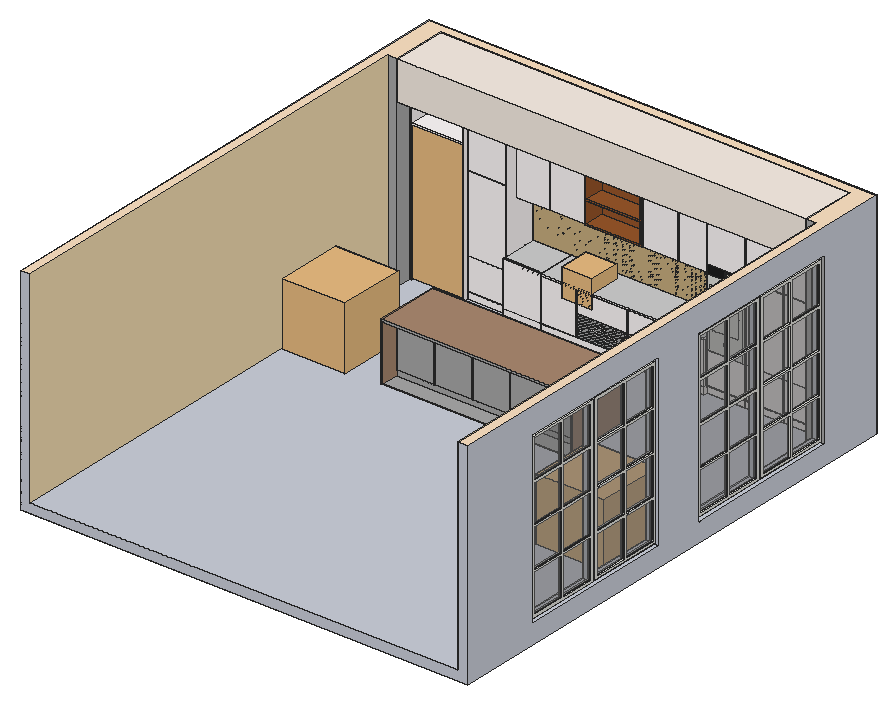
# SketchUp Ruby script. Lengths in millimetres.
U = 1.mm
M = Sketchup.active_model
def pt(a) = Geom::Point3d.new(a.map { |v| v * U })
def face(e, loops, mat)
  f = e.add_face(loops[0].map { |a| pt(a) })
  loops[1..].each { |l| e.add_face(l.map { |a| pt(a) }).erase! }
  f.material = f.back_material = mat if mat
  f
end
# faces: each face lists its corners as indices into pts; further lists are holes
def faces(e, pts, list, mat = nil) = list.each { |f| face(e, (f[0].is_a?(Array) ? f : [f]).map { |l| l.map { |i| pts[i] } }, mat) }
# xy, xz, yz: faces in a plane at the given z, y or x. An outline is a flat list of corners, or four numbers for a rectangle; further outlines are holes
def ring(l) = l.size == 4 ? [[l[0], l[1]], [l[2], l[1]], [l[2], l[3]], [l[0], l[3]]] : l.each_slice(2).to_a
def flat(e, list, mat, &to3) = list.each { |f| face(e, (f[0].is_a?(Array) ? f : [f]).map { |l| ring(l).map { |u, v| to3.(u, v) } }, mat) }
def xy(e, z, list, mat = nil) = flat(e, list, mat) { |x, y| [x, y, z] }
def xz(e, y, list, mat = nil) = flat(e, list, mat) { |x, z| [x, y, z] }
def yz(e, x, list, mat = nil) = flat(e, list, mat) { |y, z| [x, y, z] }
def lines(e, pts, list) = list.each { |a, b| e.add_line(pt(pts[a]), pt(pts[b])) }
# prism: a flat outline (further loops are holes) pulled along v
def prism(e, loops, v, mat = nil)
  f = face(e, loops, mat); d = Geom::Vector3d.new(v.map { |x| x * U })
  f.pushpull(f.normal.samedirection?(d) ? d.length : -d.length)
end
def box(e, o, s, mat = nil) = prism(e, [[o, [o[0] + s[0], o[1], o[2]], [o[0] + s[0], o[1] + s[1], o[2]], [o[0], o[1] + s[1], o[2]]]], [0, 0, s[2]], mat)
def at(x, y, z, deg = 0) = Geom::Transformation.translation(pt([x, y, z])) * Geom::Transformation.rotation(ORIGIN, Z_AXIS, deg.degrees)
def axes(o, x, y, z) = Geom::Transformation.new([*x, 0, *y, 0, *z, 0, *pt(o).to_a, 1])
def part(name) = M.definitions.add(name)
# library, detail: a bought-in or finely detailed component or shape, given as its bounding box
def library(name, o, s) = part(name).tap { |d| box(d.entities, o, s) }
def detail(e, o, s) = box(e.add_group.entities, o, s)
def put(e, d, t, mat = nil) = e.add_instance(d, t).tap { |i| i.material = mat if mat }
def group(e, t, mat = nil) = e.add_group.tap { |g| g.transformation = t; g.material = mat if mat }.entities
root = M.entities
M.materials.add("[0009_Linen]").color = [250, 240, 230]
M.materials.add("[0010_Snow]").color = [255, 250, 250]
M.materials.add("[0012_Bisque]").color = [255, 228, 196]
M.materials.add("[0034_Wheat]").color = [245, 222, 179]
M.materials.add("[0132_LightGray]").color = [169, 169, 169]
M.materials.add("[Carrera Marble]").color = [207, 207, 207]
M.materials.add("[Color M03]").color = [170, 170, 170]
M.materials.add("[Color_008]").color = [30, 30, 30]
M.materials.add("[Marble Carrara Floor Tile]").color = [204, 208, 219]
M.materials.add("[Roofing Slate Tan]").color = [200, 175, 128]
M.materials.add("[Tile Veriegated Stone]").color = [171, 137, 112]
M.materials.add("[Translucent Glass Gray]").color = [128, 128, 128]
M.materials["[Translucent Glass Gray]"].alpha = 0.5
M.materials.add("[Wood Cherry Original]").color = [152, 86, 42]
c1 = library("Untitled",[1978.1,21049.9,34.3],[1077.2,950.8,1997.1])
c2 = library("Component_3",[0,0,0],[480,480,433.8])
c3 = part("kg")
xy(c3.entities,0.03,[[[6.76,0,6.01,0.06,5.3,0.21,5.3,1.09,5.35,1.09,5.6,0.99,5.97,0.88,6.4,0.79,6.83,0.75,7.19,0.78,7.49,0.85,7.73,0.98,7.91,1.14,8.11,1.56,8.17,2.11,8.17,2.55,7.83,2.3,7.51,2.12,7.14,2.01,6.69,1.98,6.28,2.02,5.92,2.13,5.6,2.33,5.33,2.61,5.11,2.96,4.95,3.38,4.85,3.87,4.82,4.43,4.87,5.02,5,5.54,5.2,5.98,5.47,6.35,5.77,6.64,6.13,6.85,6.52,6.98,6.93,7.02,7.6,6.93,8.17,6.67,8.22,6.88,9.01,6.88,9.01,2.46,8.98,1.87,8.87,1.36,8.7,0.93,8.46,0.59,8.14,0.33,7.76,0.15,7.3,0.04],[6.87,2.75,7.21,2.79,7.55,2.88,7.88,3.04,8.17,3.25,8.17,5.99,7.59,6.2,7.06,6.27,6.76,6.24,6.49,6.15,6.26,6,6.06,5.8,5.9,5.54,5.78,5.23,5.69,4.45,5.76,3.72,5.97,3.19,6.13,3,6.34,2.86,6.58,2.78]],[0.61,1.89,0.61,8.85,1.45,8.85,1.45,4.77,3.42,6.88,4.47,6.88,2.42,4.8,4.75,1.89,3.64,1.89,1.78,4.3,1.45,3.98,1.45,1.89]])
c4 = part("12:15")
xy(c4.entities,0.1,[[2.4,0,2.1,0.1,1.9,0.2,1.7,0.4,1.7,1,1.9,1.2,2.1,1.3,2.4,1.4,4.5,1.4,4.5,9.6,2.1,9.6,1.7,10,1.7,10.6,1.9,10.8,2.1,10.9,2.4,11,5.9,11,5.9,1.4,7.3,1.4,7.3,4.6,7.5,4.8,7.7,4.9,8,5,8.2,4.9,8.5,4.8,8.6,4.6,8.7,4.3,8.7,0.7,8.6,0.4,8.5,0.2,8.2,0.1,8,0],[11.9,0,11.9,4.8,12,5.3,12.3,5.8,12.8,6.1,13.3,6.2,17.5,6.2,17.5,9.6,12.3,9.6,11.9,10,11.9,10.6,12.1,10.8,12.3,10.9,12.6,11,17.5,11,18.1,10.9,18.5,10.6,18.9,10.1,19,9.6,19,6.2,18.9,5.7,18.5,5.2,18.1,4.9,17.5,4.8,13.3,4.8,13.3,1.4,18.3,1.4,18.7,1.2,18.9,1,19,0.7,18.9,0.4,18.7,0.2,18.3,0],[33.1,0,32.8,0.1,32.6,0.2,32.4,0.4,32.4,1,32.6,1.2,32.8,1.3,33.1,1.4,35.2,1.4,35.2,9.6,32.8,9.6,32.6,9.8,32.5,10,32.4,10.3,32.5,10.6,32.6,10.8,32.8,10.9,33.1,11,36.6,11,36.6,1.4,38,1.4,38,4.6,38.2,4.8,38.4,4.9,38.7,5,39,4.9,39.2,4.8,39.3,4.6,39.4,4.3,39.4,0.7,39.3,0.4,39.2,0.2,39,0.1,38.7,0],[45.2,0,44.8,0.1,44.3,0.2,43.2,0.6,42.9,0.9,42.8,1.3,42.9,1.6,43,1.8,43.2,2,43.5,2,44,1.9,44.9,1.5,45.2,1.4,48.4,1.4,48.4,4.8,44.2,4.8,44.2,11,49.1,11,49.4,10.9,49.6,10.8,49.8,10.6,49.8,10,49.4,9.6,45.6,9.6,45.6,6.2,48.4,6.2,49,6.1,49.4,5.8,49.7,5.3,49.8,4.8,49.8,1.4,49.7,0.9,49.4,0.4,49,0.1,48.4,0],[24.7,1.8,24.3,2.2,24.3,3.9,24.5,4.2,24.7,4.3,25,4.4,26.4,4.4,26.6,4.3,26.9,4.2,27,3.9,27.1,3.7,27.1,2.5,27,2.2,26.9,2,26.7,1.8],
  [24.7,6.6,24.3,7,24.3,8.7,24.5,9,24.7,9.1,25,9.2,26.4,9.2,26.7,9.1,26.9,8.9,27.1,8.5,27.1,7.3,27,7,26.9,6.8,26.7,6.6]])
c5 = part("Siemens")
xy(c5.entities,0.1,[[3.5,0,2.8,0.1,2.2,0.6,1.8,1.2,1.7,1.8,1.7,2.2,1.9,2.4,2.1,2.5,2.4,2.6,2.7,2.5,2.9,2.4,3.1,2.2,3.1,1.7,3.4,1.4,7.3,1.4,7.3,1.6,7.2,1.8,2.1,8.4,1.8,8.9,1.7,9.4,1.8,10,2.2,10.5,2.7,10.9,3.3,11,6.9,11,7.5,10.9,8.2,10.4,8.6,9.8,8.7,9.1,8.7,8.8,8.3,8.4,7.8,8.4,7.6,8.5,7.1,9.5,6.8,9.6,3.4,9.6,3.2,9.5,3.1,9.4,3.2,9.2,8.4,2.6,8.7,2.1,8.7,1.6,8.6,1,8.3,0.5,7.8,0.1,7.3,0],[13.3,0,13.1,0.1,12.8,0.2,12.7,0.4,12.6,0.7,12.7,1,12.8,1.2,13.1,1.4,14.7,1.4,14.7,6.6,13.1,6.6,12.8,6.8,12.7,7,12.6,7.3,12.7,7.6,12.8,7.8,13.1,8,15.7,8,16,7.8,16.1,7.6,16.2,7.3,16.2,1.4,17.8,1.4,18.2,1,18.3,0.7,18.2,0.4,18.1,0.2,17.8,0.1,17.6,0],[[24.8,0,24.1,0.2,23.5,0.5,22.9,1,22.6,1.3,22.2,2.1,22.2,5.6,22.4,6.3,22.6,6.8,22.9,7.1,24.1,7.9,24.8,8,26.7,8,27.4,7.8,28.1,7.4,28.9,6.6,29.1,6.2,29.2,5.4,29.2,3.7,29.1,3.4,29,3.2,28.8,3,23.6,3,23.6,2.6,23.7,2.3,23.9,2,24.3,1.6,24.9,1.4,28.5,1.4,28.8,1.3,29,1.2,29.1,1,29.2,0.7,29.1,0.4,29,0.2,28.8,0.1,28.5,0],[23.6,4.4,27.8,4.4,27.8,5.7,27.6,6,27.2,6.3,26.9,6.5,26.6,6.6,24.9,6.6,24.3,6.4,23.7,5.8,23.6,5.5]],[33,0,32.7,0.1,32.5,0.2,32.3,0.4,32.3,7.6,32.5,7.8,32.7,7.9,33,8,33.4,7.9,33.6,7.5,34.2,7.9,34.9,8,35.3,8,35.7,7.8,36,7.6,36.3,7.3,37,7.8,37.4,8,37.7,8,38.3,7.9,38.9,7.5,39.2,7,39.4,6.4,39.6,0.7,39.5,0.4,39.4,0.2,39.1,0.1,38.9,0,38.6,0.1,38.4,0.2,38.2,0.4,38.2,0.7,38,6.1,37.9,6.5,37.7,6.6,37.4,6.5,36.6,5.8,36.6,0.4,36.4,0.2,36.2,0.1,35.9,0,35.7,0.1,35.4,0.2,35.3,0.4,35.2,0.7,35.2,6.2,35.1,6.5,34.9,6.6,34.6,6.5,33.6,5.6,33.6,0.4,33.4,0.2],[[45.3,0,44.5,0.2,44,0.5,43.3,1,43.1,1.3,42.8,1.7,42.7,2.1,42.7,5.6,42.9,6.3,43.1,6.8,43.4,7.1,44.6,7.9,45.2,8,47.2,8,47.9,7.8,48.6,7.4,49.4,6.6,49.7,5.4,49.7,3.7,49.6,3.4,49.5,3.2,49.2,3,44.1,3,44.1,2.3,44.8,1.6,45.4,1.4,49,1.4,49.2,1.3,49.5,1.2,49.6,1,49.7,0.7,49.6,0.4,49.5,0.2,49.2,0.1,49,0],[44.1,4.4,48.3,4.4,48.3,5.4,48.1,6,47.7,6.3,47.4,6.5,47.1,6.6,45.3,6.6,45,6.5,44.8,6.4,44.3,6,44.1,5.8]],
  [53.6,0,53.3,0.1,53.1,0.2,53,0.4,52.9,0.7,52.9,7.3,53,7.6,53.1,7.8,53.3,8,53.9,8,54.1,7.8,54.2,7.6,54.3,7.3,54.3,6.8,55.6,7.6,56.2,7.9,57,8,57.7,8,58.4,7.9,59.1,7.4,59.6,6.8,59.7,6,59.9,0.7,59.9,0.4,59.7,0.2,59.5,0.1,59.2,0,59,0,58.7,0.2,58.6,0.4,58.5,0.7,58.3,5.9,58.3,6.2,57.9,6.6,56.5,6.6,56.2,6.4,54.3,5.1,54.3,0.7,54.2,0.4,54.1,0.2,53.9,0.1],[65.1,0,64.4,0.1,63.8,0.4,63.3,0.9,63.1,1.3,63.2,1.5,63.3,1.8,63.9,2,64.1,1.9,64.4,1.7,64.8,1.5,65.3,1.4,68.2,1.4,68.4,1.6,68.6,1.9,68.6,2.2,68.5,2.6,68.1,2.8,64.4,4.5,63.9,4.8,63.6,5.2,63.4,5.7,63.3,6.1,63.4,6.8,63.8,7.4,64.4,7.9,65.1,8,68.3,8,69,7.9,69.6,7.5,70,7.1,70.2,6.7,70.1,6.4,70,6.2,69.7,6,69.5,6,69.2,6.1,68.6,6.5,68.3,6.6,65.2,6.6,64.8,6.5,64.7,6.2,64.8,6,65,5.8,68.7,4.2,69.2,3.8,69.6,3.4,69.9,2.8,70,2.1,69.8,1.3,69.6,0.9,69.4,0.6,68.7,0.2,67.9,0],[14.7,9.6,14.4,9.7,14.2,9.8,14.1,10.1,14,10.3,14,10.9,14.1,11.2,14.2,11.4,14.5,11.6,15.7,11.6,16,11.4,16.1,11.2,16.2,10.9,16.2,10.3,16.1,10.1,16,9.8,15.7,9.7,15.5,9.6]])
c6 = part("Naamloos")
xy(c6.entities,0,[[0,-594,550,0]])
xy(c6.entities,304,[[-14,-534,0,-514],[-14,-80,0,-60]])
xy(c6.entities,324,[[-14,-534,0,-514],[-14,-80,0,-60]])
xy(c6.entities,367.3,[[-3,-350,0,-333.4],[-3,-333.4,0,-316.8],[-3,-316.8,0,-302.6],[-3,-302.6,0,-286.7],[-3,-286.7,0,-271.3],
  [-3,-271.3,0,-257.1],[-3,-257.1,0,-244]])
xy(c6.entities,375.3,[[-3,-350,0,-333.4],[-3,-333.4,0,-316.8],[-3,-316.8,0,-302.6],[-3,-302.6,0,-286.7],[-3,-286.7,0,-271.3],
  [-3,-271.3,0,-257.1],[-3,-257.1,0,-244]])
xy(c6.entities,450,[[0,-594,550,0]])
xz(c6.entities,-594,[[0,0,550,450]])
xz(c6.entities,-534,[[-14,304,-11.4,304.3,-9,305.3,-6.9,306.9,-5.3,309,-4.3,311.4,-4,314,-4.3,316.6,-5.3,319,-6.9,321.1,-9,322.7,-11.4,323.7,-14,324,-16.6,323.7,-19,322.7,-21.1,321.1,-22.7,319,-23.7,316.6,-24,314,-23.7,311.4,-22.7,309,-21.1,306.9,-19,305.3,-16.6,304.3],[-14,304,0,324]])
xz(c6.entities,-514,[[-14,304,0,324]])
xz(c6.entities,-350,[[-3,367.3,0,375.3]])
xz(c6.entities,-244,[[-3,367.3,0,375.3]])
xz(c6.entities,-80,[[-14,304,0,324]])
xz(c6.entities,-60,[[-14,304,-16.6,304.3,-19,305.3,-21.1,306.9,-22.7,309,-23.7,311.4,-24,314,-23.7,316.6,-22.7,319,-21.1,321.1,-19,322.7,-16.6,323.7,-14,324,-11.4,323.7,-9,322.7,-6.9,321.1,-5.3,319,-4.3,316.6,-4,314,-4.3,311.4,-5.3,309,-6.9,306.9,-9,305.3,-11.4,304.3],[-14,304,0,324]])
xz(c6.entities,0,[[0,0,550,450]])
yz(c6.entities,-14,[[-534,304,-514,324],[-80,304,-60,324]])
yz(c6.entities,-6,[[-388.4,353.6,-392.8,354.2,-396.9,356,-400.3,358.7,-403,362.3,-404.6,366.4,-405.1,370.8,-404.5,375.2,-402.7,379.3,-399.9,382.8,-396.4,385.4,-392.2,387,-387.8,387.5,-383.4,386.9,-379.4,385.1,-375.9,382.4,-373.2,378.8,-371.6,374.7,-371.1,370.3,-371.8,365.9,-373.5,361.8,-376.3,358.3,-379.9,355.7,-384,354.1],[-206.2,354.2,-210.9,354.3,-215.4,355.7,-219.4,358.1,-222.7,361.6,-224.9,365.7,-226,370.3,-225.8,375,-224.5,379.5,-222,383.5,-218.6,386.7,-214.5,388.9,-209.9,390,-205.2,389.9,-200.7,388.5,-196.7,386.1,-193.5,382.6,-191.2,378.5,-190.2,373.9,-190.3,369.2,-191.6,364.7,-194.1,360.7,-197.5,357.5,-201.7,355.3]])
yz(c6.entities,-3,[[-350,367.3,-333.4,375.3],[-333.4,367.3,-316.8,375.3],[-316.8,367.3,-302.6,375.3],[-302.6,367.3,-286.7,375.3],[-286.7,367.3,-271.3,375.3],
  [-271.3,367.3,-257.1,375.3],[-257.1,367.3,-244,375.3]])
yz(c6.entities,0,[[[-594,0,-594,400,0,400,0,0,-30,0,-30,350,-564,350,-564,0],[-206.2,354.2,-201.7,355.3,-197.5,357.5,-194.1,360.7,-191.6,364.7,-190.3,369.2,-190.2,373.9,-191.2,378.5,-193.5,382.6,-196.7,386.1,-200.7,388.5,-205.2,389.9,-209.9,390,-214.5,388.9,-218.6,386.7,-222,383.5,-224.5,379.5,-225.8,375,-226,370.3,-224.9,365.7,-222.7,361.6,-219.4,358.1,-215.4,355.7,-210.9,354.3],[-388.4,353.6,-384,354.1,-379.9,355.7,-376.3,358.3,-373.5,361.8,-371.8,365.9,-371.1,370.3,-371.6,374.7,-373.2,378.8,-375.9,382.4,-379.4,385.1,-383.4,386.9,-387.8,387.5,-392.2,387,-396.4,385.4,-399.9,382.8,-402.7,379.3,-404.5,375.2,-405.1,370.8,-404.6,366.4,-403,362.3,-400.3,358.7,-396.9,356,-392.8,354.2],[-350,367.3,-244,375.3],[-249.2,382.1,-248.5,382.2,-247.7,382.5,-247.1,383,-246.6,383.6,-246.3,384.3,-246.2,385.1,-246.3,385.9,-246.6,386.6,-247.1,387.2,-247.7,387.7,-248.5,388,-249.2,388.1,-250,388,-250.7,387.7,-251.4,387.2,-251.8,386.6,-252.1,385.9,-252.2,385.1,-252.1,384.3,-251.8,383.6,-251.4,383,-250.7,382.5,-250,382.2],[-309.9,381.3,-309.1,381.4,-308.4,381.7,-307.8,382.1,-307.3,382.8,-307,383.5,-306.9,384.3,-307,385,-307.3,385.8,-307.8,386.4,-308.4,386.9,-309.1,387.2,-309.9,387.3,-310.7,387.2,-311.4,386.9,-312,386.4,-312.5,385.8,-312.8,385,-312.9,384.3,-312.8,383.5,-312.5,382.8,-312,382.1,-311.4,381.7,-310.7,381.4]],[[-564,0,-30,350],[-497,113,-97,263],[-534,304,-514,324],[-80,304,-60,324]],[-497,113,-97,263],[-309.9,381.3,-310.7,381.4,-311.4,381.7,-312,382.1,-312.5,382.8,-312.8,383.5,-312.9,384.3,-312.8,385,-312.5,385.8,-312,386.4,-311.4,386.9,-310.7,387.2,-309.9,387.3,-309.1,387.2,-308.4,386.9,-307.8,386.4,-307.3,385.8,-307,385,-306.9,384.3,-307,383.5,-307.3,382.8,-307.8,382.1,-308.4,381.7,-309.1,381.4],[-249.2,382.1,-250,382.2,-250.7,382.5,-251.4,383,-251.8,383.6,-252.1,384.3,-252.2,385.1,-252.1,385.9,-251.8,386.6,-251.4,387.2,-250.7,387.7,-250,388,-249.2,388.1,-248.5,388,-247.7,387.7,-247.1,387.2,-246.6,386.6,-246.3,385.9,-246.2,385.1,-246.3,384.3,-246.6,383.6,-247.1,383,-247.7,382.5,-248.5,382.2]])
yz(c6.entities,0,[[-594,400,0,450]],"[Color_008]")
yz(c6.entities,550,[[-594,0,0,450]])
p = [[-14,-534,304],[-16.6,-534,304.3],[-16.6,-60,304.3],[-14,-60,304],[-14,-80,304],[-11.4,-534,304.3],
  [-11.4,-60,304.3],[-19,-534,305.3],[-19,-60,305.3],[-9,-534,305.3],[-9,-60,305.3],[-21.1,-534,306.9],
  [-21.1,-60,306.9],[-6.9,-534,306.9],[-6.9,-60,306.9],[-22.7,-534,309],[-22.7,-60,309],[-5.3,-534,309],
  [-5.3,-60,309],[-23.7,-534,311.4],[-23.7,-60,311.4],[-4.3,-534,311.4],[-4.3,-60,311.4],[-24,-534,314],
  [-24,-60,314],[-4,-534,314],[-4,-60,314],[-23.7,-534,316.6],[-23.7,-60,316.6],[-4.3,-534,316.6],
  [-4.3,-60,316.6],[-22.7,-534,319],[-22.7,-60,319],[-5.3,-534,319],[-5.3,-60,319],[-21.1,-534,321.1],
  [-21.1,-60,321.1],[-6.9,-534,321.1],[-6.9,-60,321.1],[-19,-534,322.7],[-19,-60,322.7],[-9,-534,322.7],
  [-9,-60,322.7],[-16.6,-534,323.7],[-16.6,-60,323.7],[-11.4,-534,323.7],[-11.4,-60,323.7],[-14,-534,324],
  [-14,-80,324],[-14,-60,324],[0,-388.4,353.6],[0,-392.8,354.2],[-6,-392.8,354.2],[-6,-388.4,353.6],
  [0,-384,354.1],[-6,-384,354.1],[0,-379.9,355.7],[-6,-379.9,355.7],[0,-396.9,356],[-6,-396.9,356],
  [0,-206.2,354.2],[0,-210.9,354.3],[-6,-210.9,354.3],[-6,-206.2,354.2],[0,-201.7,355.3],[-6,-201.7,355.3],
  [0,-215.4,355.7],[-6,-215.4,355.7],[0,-197.5,357.5],[-6,-197.5,357.5],[0,-376.3,358.3],[-6,-376.3,358.3],
  [0,-219.4,358.1],[-6,-219.4,358.1],[0,-400.3,358.7],[-6,-400.3,358.7],[0,-194.1,360.7],[-6,-194.1,360.7],
  [0,-222.7,361.6],[-6,-222.7,361.6],[0,-373.5,361.8],[-6,-373.5,361.8],[0,-403,362.3],[-6,-403,362.3],
  [0,-191.6,364.7],[-6,-191.6,364.7],[0,-224.9,365.7],[-6,-224.9,365.7],[0,-371.8,365.9],[-6,-371.8,365.9],
  [0,-404.6,366.4],[-6,-404.6,366.4],[0,-190.3,369.2],[-6,-190.3,369.2],[0,-226,370.3],[-6,-226,370.3],
  [0,-371.1,370.3],[-6,-371.1,370.3],[0,-405.1,370.8],[-6,-405.1,370.8],[0,-190.2,373.9],[-6,-190.2,373.9],
  [0,-371.6,374.7],[-6,-371.6,374.7],[0,-225.8,375],[-6,-225.8,375],[0,-404.5,375.2],[-6,-404.5,375.2],
  [0,-191.2,378.5],[-6,-191.2,378.5],[0,-373.2,378.8],[-6,-373.2,378.8],[0,-224.5,379.5],[-6,-224.5,379.5],
  [0,-402.7,379.3],[-6,-402.7,379.3],[0,-193.5,382.6],[-6,-193.5,382.6],[0,-375.9,382.4],[-6,-375.9,382.4],
  [0,-399.9,382.8],[-6,-399.9,382.8],[0,-222,383.5],[-6,-222,383.5],[0,-379.4,385.1],[-6,-379.4,385.1],
  [0,-196.7,386.1],[-6,-196.7,386.1],[0,-396.4,385.4],[-6,-396.4,385.4],[0,-218.6,386.7],[-6,-218.6,386.7],
  [0,-383.4,386.9],[-6,-383.4,386.9],[0,-392.2,387],[-6,-392.2,387],[0,-200.7,388.5],[-6,-200.7,388.5],
  [0,-214.5,388.9],[-6,-214.5,388.9],[0,-387.8,387.5],[-6,-387.8,387.5],[0,-205.2,389.9],[-6,-205.2,389.9],
  [0,-209.9,390],[-6,-209.9,390],[0,-260.1,384.4],[0,-266.1,384.4],[0,-275.9,384.4],[0,-281.9,384.4],
  [0,-279.1,381.9],[0,-279.1,386.9],[0,-309.9,387.3],[0,-309.9,384.3],[0,-307.9,384.3]]
faces(c6.entities,p,[[0,1,2,3,4],[5,0,4,3,6],[1,7,8,2],[9,5,6,10],[7,11,12,8],[13,9,10,14],[11,15,16,12],[17,13,14,18],
  [15,19,20,16],[21,17,18,22],[19,23,24,20],[25,21,22,26],[23,27,28,24],[29,25,26,30],[27,31,32,28],[33,29,30,34],
  [31,35,36,32],[37,33,34,38],[35,39,40,36],[41,37,38,42],[39,43,44,40],[45,41,42,46],[43,47,48,49,44],[47,45,46,49,48],
  [50,51,52,53],[54,50,53,55],[56,54,55,57],[51,58,59,52],[60,61,62,63],[64,60,63,65],[61,66,67,62],[68,64,65,69],
  [70,56,57,71],[66,72,73,67],[58,74,75,59],[76,68,69,77],[72,78,79,73],[80,70,71,81],[74,82,83,75],[84,76,77,85],
  [78,86,87,79],[88,80,81,89],[82,90,91,83],[92,84,85,93],[86,94,95,87],[96,88,89,97],[90,98,99,91],[100,92,93,101],
  [102,96,97,103],[94,104,105,95],[98,106,107,99],[108,100,101,109],[110,102,103,111],[104,112,113,105],[106,114,115,107],[116,108,109,117],
  [118,110,111,119],[114,120,121,115],[112,122,123,113],[124,118,119,125],[126,116,117,127],[120,128,129,121],[122,130,131,123],[132,124,125,133],
  [128,134,135,129],[136,126,127,137],[130,138,139,131],[140,132,133,141],[134,140,141,135],[142,136,137,143],[138,144,145,139],[144,142,143,145]])
lines(c6.entities,p,[[146,147],[148,149],[150,151],[152,153],[153,154]])
put(c6.entities,c3,axes([0,-289.7,380.2],[0,-1,0],[0,0,1],[-1,0,0]))
put(c6.entities,c4,axes([0,-270.7,426.7],[0,-1,0],[0,0,1],[-1,0,0]))
put(c6.entities,c5,axes([0,-261.9,52.3],[0,-1,0],[0,0,1],[-1,0,0]))
c7 = library("plant",[-542,-691.1,-9.7],[1064.4,1045.2,990])
xy(root,890,[[2650,7330,3150,7730]])
xy(root,900,[[2650,7330,3150,7730]])
xy(root,910,[[2650,7330,3150,7730]])
xy(root,920,[[[2650,7330,3150,7730],[2677.7,7357.7,3122.3,7702.3]],[2677.7,7357.7,3122.3,7702.3]])
xy(root,950,[[1750.2,7850,4900,8510]])
xy(root,1700,[[1750.2,7850,4900,8510]])
xz(root,7250,[[2900,250,4300,585]],"[Color M03]")
xz(root,7330,[[2650,890,3150,900],[2650,900,3150,910],[2650,910,3150,920]])
xz(root,7730,[[2650,890,3150,900],[2650,900,3150,910],[2650,910,3150,920]])
xz(root,7850,[[1750.2,950,4900,1700]],"[Roofing Slate Tan]")
xz(root,8510,[[1750.2,950,4900,1700]])
yz(root,1750.2,[[7850,950,8510,1700]])
yz(root,2650,[[7330,890,7730,900],[7330,900,7730,910],[7330,910,7730,920]])
yz(root,3150,[[7330,890,7730,900],[7330,900,7730,910],[7330,910,7730,920]])
yz(root,4900,[[7850,950,8510,1700]])
p = [[1750,7250,250],[2350,7250,250]]
lines(root,p,[[0,1]])
put(root,c1,axes([-1257.1,-2186.7,142.2],[0.77804,0,0],[0,0.4483,0],[0,0,1.07208]))
put(root,c2,at(2670,7730,721.8,-90))
put(root,c6,axes([4901,7310,755],[0,0.57,0],[-1,0,0],[0,0,2.66667]))
put(root,c7,at(621.6,5612.8,150))
put(root,c7,at(6172.1,3743.6,159.7))
g1 = group(root,at(6925,4550,350))
xy(g1,0,[[0,-3250,50,-2075],[0,-2025,50,-850],[0,0,50,1175]])
xy(g1,30,[[0,-3220,30,-2672.5],[30,-3220,50,-2672.5],[0,-2652.5,30,-2105],[30,-2652.5,50,-2105],[0,-1995,30,-1447.5],
  [30,-1995,50,-1447.5],[0,-1427.5,30,-880],[30,-1427.5,50,-880],[0,30,30,577.5],[30,30,50,577.5],
  [0,597.5,30,1145],[30,597.5,50,1145]])
xy(g1,637.5,[[0,-3220,30,-2672.5],[30,-3220,50,-2672.5],[0,-2652.5,30,-2105],[30,-2652.5,50,-2105],[0,-1995,30,-1447.5],
  [30,-1995,50,-1447.5],[0,-1427.5,30,-880],[30,-1427.5,50,-880],[0,30,30,577.5],[30,30,50,577.5],
  [0,597.5,30,1145],[30,597.5,50,1145]])
xy(g1,657.5,[[0,-3220,30,-2672.5],[30,-3220,50,-2672.5],[0,-2652.5,30,-2105],[30,-2652.5,50,-2105],[0,-1995,30,-1447.5],
  [30,-1995,50,-1447.5],[0,-1427.5,30,-880],[30,-1427.5,50,-880],[0,30,30,577.5],[30,30,50,577.5],
  [0,597.5,30,1145],[30,597.5,50,1145]])
xy(g1,1265,[[0,-3220,30,-2672.5],[30,-3220,50,-2672.5],[0,-2652.5,30,-2105],[30,-2652.5,50,-2105],[0,-1995,30,-1447.5],
  [30,-1995,50,-1447.5],[0,-1427.5,30,-880],[30,-1427.5,50,-880],[0,30,30,577.5],[30,30,50,577.5],
  [0,597.5,30,1145],[30,597.5,50,1145]])
xy(g1,1285,[[0,-3220,30,-2672.5],[30,-3220,50,-2672.5],[0,-2652.5,30,-2105],[30,-2652.5,50,-2105],[0,-1995,30,-1447.5],
  [30,-1995,50,-1447.5],[0,-1427.5,30,-880],[30,-1427.5,50,-880],[0,30,30,577.5],[30,30,50,577.5],
  [0,597.5,30,1145],[30,597.5,50,1145]])
xy(g1,1892.5,[[0,-3220,30,-2672.5],[30,-3220,50,-2672.5],[0,-2652.5,30,-2105],[30,-2652.5,50,-2105],[0,-1995,30,-1447.5],
  [30,-1995,50,-1447.5],[0,-1427.5,30,-880],[30,-1427.5,50,-880],[0,30,30,577.5],[30,30,50,577.5],
  [0,597.5,30,1145],[30,597.5,50,1145]])
xy(g1,1912.5,[[0,-3220,30,-2672.5],[30,-3220,50,-2672.5],[0,-2652.5,30,-2105],[30,-2652.5,50,-2105],[0,-1995,30,-1447.5],
  [30,-1995,50,-1447.5],[0,-1427.5,30,-880],[30,-1427.5,50,-880],[0,30,30,577.5],[30,30,50,577.5],
  [0,597.5,30,1145],[30,597.5,50,1145]])
xy(g1,2520,[[0,-3220,30,-2672.5],[30,-3220,50,-2672.5],[0,-2652.5,30,-2105],[30,-2652.5,50,-2105],[0,-1995,30,-1447.5],
  [30,-1995,50,-1447.5],[0,-1427.5,30,-880],[30,-1427.5,50,-880],[0,30,30,577.5],[30,30,50,577.5],
  [0,597.5,30,1145],[30,597.5,50,1145]])
xy(g1,2550,[[0,-3250,50,-2075],[0,-2025,50,-850],[0,0,50,1175]])
xz(g1,-3250,[[0,0,50,2550]])
xz(g1,-3220,[[0,30,30,637.5],[30,30,50,637.5],[0,657.5,30,1265],[30,657.5,50,1265],[0,1285,30,1892.5],
  [30,1285,50,1892.5],[0,1912.5,30,2520],[30,1912.5,50,2520]])
xz(g1,-2672.5,[[0,30,30,637.5],[30,30,50,637.5],[0,657.5,30,1265],[30,657.5,50,1265],[0,1285,30,1892.5],
  [30,1285,50,1892.5],[0,1912.5,30,2520],[30,1912.5,50,2520]])
xz(g1,-2652.5,[[0,30,30,637.5],[30,30,50,637.5],[0,657.5,30,1265],[30,657.5,50,1265],[0,1285,30,1892.5],
  [30,1285,50,1892.5],[0,1912.5,30,2520],[30,1912.5,50,2520]])
xz(g1,-2105,[[0,30,30,637.5],[30,30,50,637.5],[0,657.5,30,1265],[30,657.5,50,1265],[0,1285,30,1892.5],
  [30,1285,50,1892.5],[0,1912.5,30,2520],[30,1912.5,50,2520]])
xz(g1,-2075,[[0,0,50,2550]])
xz(g1,-2025,[[0,0,50,2550]])
xz(g1,-1995,[[0,30,30,637.5],[30,30,50,637.5],[0,657.5,30,1265],[30,657.5,50,1265],[0,1285,30,1892.5],
  [30,1285,50,1892.5],[0,1912.5,30,2520],[30,1912.5,50,2520]])
xz(g1,-1447.5,[[0,30,30,637.5],[30,30,50,637.5],[0,657.5,30,1265],[30,657.5,50,1265],[0,1285,30,1892.5],
  [30,1285,50,1892.5],[0,1912.5,30,2520],[30,1912.5,50,2520]])
xz(g1,-1427.5,[[0,30,30,637.5],[30,30,50,637.5],[0,657.5,30,1265],[30,657.5,50,1265],[0,1285,30,1892.5],
  [30,1285,50,1892.5],[0,1912.5,30,2520],[30,1912.5,50,2520]])
xz(g1,-880,[[0,30,30,637.5],[30,30,50,637.5],[0,657.5,30,1265],[30,657.5,50,1265],[0,1285,30,1892.5],
  [30,1285,50,1892.5],[0,1912.5,30,2520],[30,1912.5,50,2520]])
xz(g1,-850,[[0,0,50,2550]])
xz(g1,0,[[0,0,50,2550]])
xz(g1,30,[[0,30,30,637.5],[30,30,50,637.5],[0,657.5,30,1265],[30,657.5,50,1265],[0,1285,30,1892.5],
  [30,1285,50,1892.5],[0,1912.5,30,2520],[30,1912.5,50,2520]])
xz(g1,577.5,[[0,30,30,637.5],[30,30,50,637.5],[0,657.5,30,1265],[30,657.5,50,1265],[0,1285,30,1892.5],
  [30,1285,50,1892.5],[0,1912.5,30,2520],[30,1912.5,50,2520]])
xz(g1,597.5,[[0,30,30,637.5],[30,30,50,637.5],[0,657.5,30,1265],[30,657.5,50,1265],[0,1285,30,1892.5],
  [30,1285,50,1892.5],[0,1912.5,30,2520],[30,1912.5,50,2520]])
xz(g1,1145,[[0,30,30,637.5],[30,30,50,637.5],[0,657.5,30,1265],[30,657.5,50,1265],[0,1285,30,1892.5],
  [30,1285,50,1892.5],[0,1912.5,30,2520],[30,1912.5,50,2520]])
xz(g1,1175,[[0,0,50,2550]])
yz(g1,0,[[[-3250,0,-2075,2550],[-2652.5,30,-2105,637.5],[-3220,1912.5,-2672.5,2520],[-2652.5,657.5,-2105,1265],[-3220,30,-2672.5,637.5],[-2652.5,1285,-2105,1892.5],[-2652.5,1912.5,-2105,2520],[-3220,1285,-2672.5,1892.5],[-3220,657.5,-2672.5,1265]],[[-2025,0,-850,2550],[-1995,1912.5,-1447.5,2520],[-1427.5,30,-880,637.5],[-1427.5,657.5,-880,1265],[-1995,30,-1447.5,637.5],[-1427.5,1912.5,-880,2520],[-1427.5,1285,-880,1892.5],[-1995,1285,-1447.5,1892.5],[-1995,657.5,-1447.5,1265]],[[0,0,1175,2550],[30,1912.5,577.5,2520],[597.5,30,1145,637.5],[597.5,657.5,1145,1265],[597.5,1912.5,1145,2520],[597.5,1285,1145,1892.5],[30,1285,577.5,1892.5],[30,30,577.5,637.5],[30,657.5,577.5,1265]]])
yz(g1,30,[[-3220,30,-2672.5,637.5],[-2652.5,30,-2105,637.5],[-1995,30,-1447.5,637.5],[-1427.5,30,-880,637.5],[30,30,577.5,637.5],
  [597.5,30,1145,637.5],[-3220,657.5,-2672.5,1265],[-2652.5,657.5,-2105,1265],[-1995,657.5,-1447.5,1265],[-1427.5,657.5,-880,1265],
  [30,657.5,577.5,1265],[597.5,657.5,1145,1265],[-3220,1285,-2672.5,1892.5],[-2652.5,1285,-2105,1892.5],[-1995,1285,-1447.5,1892.5],
  [-1427.5,1285,-880,1892.5],[30,1285,577.5,1892.5],[597.5,1285,1145,1892.5],[-3220,1912.5,-2672.5,2520],[-2652.5,1912.5,-2105,2520],
  [-1995,1912.5,-1447.5,2520],[-1427.5,1912.5,-880,2520],[30,1912.5,577.5,2520],[597.5,1912.5,1145,2520]],"[Translucent Glass Gray]")
yz(g1,50,[[[-3250,0,-2075,2550],[-2652.5,30,-2105,637.5],[-3220,1912.5,-2672.5,2520],[-2652.5,657.5,-2105,1265],[-3220,30,-2672.5,637.5],[-2652.5,1285,-2105,1892.5],[-2652.5,1912.5,-2105,2520],[-3220,1285,-2672.5,1892.5],[-3220,657.5,-2672.5,1265]],[[-2025,0,-850,2550],[-1995,1912.5,-1447.5,2520],[-1427.5,30,-880,637.5],[-1427.5,657.5,-880,1265],[-1995,30,-1447.5,637.5],[-1427.5,1912.5,-880,2520],[-1427.5,1285,-880,1892.5],[-1995,1285,-1447.5,1892.5],[-1995,657.5,-1447.5,1265]],[[0,0,1175,2550],[30,1912.5,577.5,2520],[597.5,30,1145,637.5],[597.5,1285,1145,1892.5],[597.5,657.5,1145,1265],[30,1285,577.5,1892.5],[30,30,577.5,637.5],[597.5,1912.5,1145,2520],[30,657.5,577.5,1265]]])
g2 = group(root,at(6925,5775,350))
xy(g2,0,[[0,0,50,1175]])
xy(g2,30,[[0,30,30,577.5],[30,30,50,577.5],[0,597.5,30,1145],[30,597.5,50,1145]])
xy(g2,637.5,[[0,30,30,577.5],[30,30,50,577.5],[0,597.5,30,1145],[30,597.5,50,1145]])
xy(g2,657.5,[[0,30,30,577.5],[30,30,50,577.5],[0,597.5,30,1145],[30,597.5,50,1145]])
xy(g2,1265,[[0,30,30,577.5],[30,30,50,577.5],[0,597.5,30,1145],[30,597.5,50,1145]])
xy(g2,1285,[[0,30,30,577.5],[30,30,50,577.5],[0,597.5,30,1145],[30,597.5,50,1145]])
xy(g2,1892.5,[[0,30,30,577.5],[30,30,50,577.5],[0,597.5,30,1145],[30,597.5,50,1145]])
xy(g2,1912.5,[[0,30,30,577.5],[30,30,50,577.5],[0,597.5,30,1145],[30,597.5,50,1145]])
xy(g2,2520,[[0,30,30,577.5],[30,30,50,577.5],[0,597.5,30,1145],[30,597.5,50,1145]])
xy(g2,2550,[[0,0,50,1175]])
xz(g2,0,[[0,0,50,2550]])
xz(g2,30,[[0,30,30,637.5],[30,30,50,637.5],[0,657.5,30,1265],[30,657.5,50,1265],[0,1285,30,1892.5],
  [30,1285,50,1892.5],[0,1912.5,30,2520],[30,1912.5,50,2520]])
xz(g2,577.5,[[0,30,30,637.5],[30,30,50,637.5],[0,657.5,30,1265],[30,657.5,50,1265],[0,1285,30,1892.5],
  [30,1285,50,1892.5],[0,1912.5,30,2520],[30,1912.5,50,2520]])
xz(g2,597.5,[[0,30,30,637.5],[30,30,50,637.5],[0,657.5,30,1265],[30,657.5,50,1265],[0,1285,30,1892.5],
  [30,1285,50,1892.5],[0,1912.5,30,2520],[30,1912.5,50,2520]])
xz(g2,1145,[[0,30,30,637.5],[30,30,50,637.5],[0,657.5,30,1265],[30,657.5,50,1265],[0,1285,30,1892.5],
  [30,1285,50,1892.5],[0,1912.5,30,2520],[30,1912.5,50,2520]])
xz(g2,1175,[[0,0,50,2550]])
yz(g2,0,[[[0,0,1175,2550],[597.5,30,1145,637.5],[597.5,657.5,1145,1265],[597.5,1285,1145,1892.5],[597.5,1912.5,1145,2520],[30,1912.5,577.5,2520],[30,30,577.5,637.5],[30,1285,577.5,1892.5],[30,657.5,577.5,1265]]])
yz(g2,30,[[30,30,577.5,637.5],[597.5,30,1145,637.5],[30,657.5,577.5,1265],[597.5,657.5,1145,1265],[30,1285,577.5,1892.5],
  [597.5,1285,1145,1892.5],[30,1912.5,577.5,2520],[597.5,1912.5,1145,2520]],"[Translucent Glass Gray]")
yz(g2,50,[[[0,0,1175,2550],[597.5,30,1145,637.5],[597.5,657.5,1145,1265],[597.5,1285,1145,1892.5],[597.5,1912.5,1145,2520],[30,1912.5,577.5,2520],[30,30,577.5,637.5],[30,1285,577.5,1892.5],[30,657.5,577.5,1265]]])
g3 = group(root,at(6100,7850,150),"[0010_Snow]")
xy(g3,-30,[[-4450,-2850,-1450,-1850]])
xy(g3,0,[[-4350,-600,-3750,0],[-4950,-540,-4350,0],[-1200,-540,-600,0],[-600,-540,0,0],[0,-540,600,0]])
xy(g3,0,[[-4420,-2850,-1480,-2580]],"[0132_LightGray]")
xy(g3,77.9,[[-4420,-2580,-1480,-2560]])
xy(g3,82.9,[[-4415,-2580,-4401.6,-2560],[-4401.6,-2580,-3837,-2560],[-3827,-2580,-3249,-2560],[-3239,-2580,-2661,-2560],[-2651,-2580,-2073,-2560],
  [-2063,-2580,-1485,-2560]])
xy(g3,100,[[-4950,-540,-4350,-520],[-1200,-540,-600,-520],[-600,-540,0,-520],[0,-540,600,-520]])
xy(g3,105,[[-4945,-540,-4355,-520],[-1195,-540,-605,-520],[-595,-540,-5,-520],[5,-540,595,-520]])
xy(g3,595,[[-4945,-540,-4355,-520],[-1195,-540,-605,-520],[-595,-540,-5,-520],[5,-540,595,-520]])
xy(g3,605,[[-4945,-540,-4355,-520],[-595,-540,-5,-520],[5,-540,595,-520],[-1195,-520,-605,-240]])
xy(g3,865,[[-4415,-2580,-3837,-2560],[-3827,-2580,-3249,-2560],[-3239,-2580,-2661,-2560],[-2651,-2580,-2073,-2560],[-2063,-2580,-1485,-2560]])
xy(g3,870,[[-4420,-2850,-1480,-2560]])
xy(g3,900,[[-4450,-2850,-1450,-1850]],"[Tile Veriegated Stone]")
xy(g3,1795,[[-4945,-540,-4355,-520],[-595,-540,-5,-520],[5,-540,595,-520],[-1195,-520,-605,-240]])
xy(g3,1805,[[-4945,-540,-4355,-520],[-1195,-540,-605,-520],[-595,-540,-5,-520],[5,-540,595,-520]])
xy(g3,2595,[[-4945,-540,-4355,-520],[-1195,-540,-605,-520],[-595,-540,-5,-520],[5,-540,595,-520]])
xy(g3,2600,[[-4950,-520,-4350,0],[-1200,-520,-600,0],[-600,-520,0,0],[0,-520,600,0]])
xz(g3,-2850,[[[-4450,-30,-1450,900],[-4420,0,-1480,870]]],"[0132_LightGray]")
xz(g3,-2580,[[-4420,0,-1480,77.9],[-4415,82.9,-3837,865],[-3827,82.9,-3249,865],[-3239,82.9,-2661,865],[-2651,82.9,-2073,865],
  [-2063,82.9,-1485,865]],"[0132_LightGray]")
xz(g3,-2560,[[[-4420,77.9,-1480,870],[-3239,82.9,-2661,865],[-2063,82.9,-1485,865],[-4415,82.9,-3837,865],[-3827,82.9,-3249,865],[-2651,82.9,-2073,865]]])
xz(g3,-1850,[[[-4450,-30,-1450,900],[-4420,0,-1480,870]],[-4420,0,-1480,870]])
xz(g3,-540,[[-4950,0,-4350,100],[-1200,0,-600,100],[-600,0,0,100],[0,0,600,100],[-4945,105,-4355,595],
  [-1195,105,-605,595],[-595,105,-5,595],[5,105,595,595],[-4945,605,-4355,1795],[-595,605,-5,1795],
  [5,605,595,1795],[-4945,1805,-4355,2595],[-1195,1805,-605,2595],[-595,1805,-5,2595],[5,1805,595,2595]])
xz(g3,-520,[[[-4950,100,-4350,2600],[-4945,605,-4355,1795],[-4945,1805,-4355,2595],[-4945,105,-4355,595]],[[-1200,100,-600,2600],[-1195,605,-605,1795],[-1195,1805,-605,2595],[-1195,105,-605,595]],[[-600,100,0,2600],[-595,605,-5,1795],[-595,1805,-5,2595],[-595,105,-5,595]],[[0,100,600,2600],[5,605,595,1795],[5,1805,595,2595],[5,105,595,595]]])
xz(g3,-240,[[-1195,605,-605,1795]])
xz(g3,0,[[-4950,0,-4350,2600],[-1200,0,-600,2600],[-600,0,0,2600],[0,0,600,2600]])
yz(g3,-4950,[[-540,0,-540,100,-520,100,-520,2600,0,2600,0,0]])
yz(g3,-4945,[[-540,105,-520,595],[-540,605,-520,1795],[-540,1805,-520,2595]])
yz(g3,-4450,[[-2850,-30,-1850,900]],"[Tile Veriegated Stone]")
yz(g3,-4420,[[-2850,0,-2580,0,-2580,77.9,-2560,77.9,-2560,870,-2850,870]],"[Tile Veriegated Stone]")
yz(g3,-4415,[[-2580,82.9,-2560,865]])
yz(g3,-4355,[[-540,105,-520,595],[-540,605,-520,1795],[-540,1805,-520,2595]])
yz(g3,-4350,[[-540,0,0,0,0,2600,-520,2600,-520,100,-540,100]])
yz(g3,-3837,[[-2580,82.9,-2560,865]])
yz(g3,-3827,[[-2580,82.9,-2560,865]])
yz(g3,-3249,[[-2580,82.9,-2560,865]])
yz(g3,-3239,[[-2580,82.9,-2560,865]])
yz(g3,-2661,[[-2580,82.9,-2560,865]])
yz(g3,-2651,[[-2580,82.9,-2560,865]])
yz(g3,-2073,[[-2580,82.9,-2560,865]])
yz(g3,-2063,[[-2580,82.9,-2560,865]])
yz(g3,-1485,[[-2580,82.9,-2560,865]])
yz(g3,-1480,[[-2850,0,-2850,870,-2560,870,-2560,77.9,-2580,77.9,-2580,0]],"[Tile Veriegated Stone]")
yz(g3,-1450,[[-2850,-30,-1850,900]],"[Tile Veriegated Stone]")
yz(g3,-1200,[[-540,0,-540,100,-520,100,-520,2600,0,2600,0,0]])
yz(g3,-1195,[[-540,105,-520,595],[-520,605,-240,1795],[-540,1805,-520,2595]])
yz(g3,-605,[[-540,105,-520,595],[-520,605,-240,1795],[-540,1805,-520,2595]])
yz(g3,-600,[[-540,0,-540,100,-520,100,-520,2600,0,2600,0,0]])
yz(g3,-595,[[-540,105,-520,595],[-540,605,-520,1795],[-540,1805,-520,2595]])
yz(g3,-5,[[-540,105,-520,595],[-540,605,-520,1795],[-540,1805,-520,2595]])
yz(g3,0,[[-540,0,-540,100,-520,100,-520,2600,0,2600,0,0]])
yz(g3,5,[[-540,105,-520,595],[-540,605,-520,1795],[-540,1805,-520,2595]])
yz(g3,595,[[-540,105,-520,595],[-540,605,-520,1795],[-540,1805,-520,2595]])
yz(g3,600,[[-540,0,-540,100,-520,100,-520,2600,0,2600,0,0]])
p = [[-11365.2,-9203.9,2595],[-11365.2,-9183.9,2595],[-7404.5,-12526.7,2595],[-7404.5,-12506.7,2595],[-11511.2,-9318.1,2595],[-11511.2,-9298.1,2595],
  [-12101.2,-9318.1,2595],[-12101.2,-9298.1,2595],[-11501.2,-9318.1,2595],[-11501.2,-9298.1,2595],[-1480,-2580,77.9],[-1461.6,-2580,77.9]]
lines(g3,p,[[0,1],[2,3],[4,5],[6,7],[8,9],[10,11]])
g4 = group(g3,at(-5800,0,0))
xy(g4,0,[[0,-600,0,0,850,0,850,-600,820,-600,820,-20,30,-20,30,-600]])
xy(g4,2170,[[30,-600,820,-20]])
xy(g4,2200,[[30,-600,820,-20]])
xy(g4,2570,[[30,-600,820,-20]])
xy(g4,2600,[[0,-600,850,0]])
xz(g4,-600,[[0,0,30,0,30,2570,820,2570,820,0,850,0,850,2600,0,2600],[30,2170,820,2200]])
xz(g4,-20,[[30,0,820,2170],[30,2200,820,2570]])
xz(g4,0,[[0,0,850,2600]])
yz(g4,0,[[-600,0,0,2600]])
yz(g4,30,[[-600,0,-20,2170],[-600,2200,-20,2570]])
yz(g4,820,[[-600,0,-20,2170],[-600,2200,-20,2570]])
yz(g4,850,[[-600,0,0,2600]])
g5 = group(g3,at(-4349.8,0,800))
xz(g5,0,[[0,0,3149.8,750]])
g6 = group(g3,at(-5800,0,2600),"[0009_Linen]")
prism(g6,[[[6400,0,0],[5800,0,0],[5200,0,0],[4600,0,0],[1450,0,0],[850,0,0],[0,0,0],[0,0,600],[6400,0,600]]],[0,-850,0])
g7 = group(root,at(4300,7850,1700),"[0010_Snow]")
xy(g7,0,[[-2560,-330,-2015,0],[-2015,-330,-2005,0],[-2005,-330,-1460,0],[-575,-330,0,0],[0,-330,600,0]])
xy(g7,5,[[-2555,-350,-2015,-330],[-2010,-350,-1470,-330],[-555,-350,-5,-330],[5,-350,595,-330]])
xy(g7,1045,[[-2555,-350,-2015,-330],[-2010,-350,-1470,-330],[-555,-350,-5,-330],[5,-350,595,-330]])
xy(g7,1050,[[-2560,-330,-2015,0],[-2015,-330,-2005,0],[-2005,-330,-1460,0],[-575,-330,0,0],[0,-330,600,0]])
xz(g7,-350,[[-2555,5,-2015,1045],[-2010,5,-1470,1045],[-555,5,-5,1045],[5,5,595,1045]])
xz(g7,-330,[[-2560,0,-2015,0,-2015,5,-2555,5,-2555,1045,-2015,1045,-2015,1050,-2560,1050],[-2015,0,-2005,5],[-2005,0,-1460,5],[-575,0,0,0,0,1050,-575,1050,-575,1045,-5,1045,-5,5,-575,5],[[0,0,600,1050],[5,5,595,1045]],
  [-2015,5,-2010,1045],[-2010,5,-2005,1045],[-1470,5,-1460,1045],[-575,5,-555,1045],[-2015,1045,-2005,1050],
  [-2005,1045,-1460,1050]])
xz(g7,0,[[-2560,0,-2015,1050],[-2015,0,-2005,1050],[-2005,0,-1460,1050],[-575,0,0,1050],[0,0,600,1050]])
yz(g7,-2560,[[-330,0,0,1050]])
yz(g7,-2555,[[-350,5,-330,1045]])
yz(g7,-2015,[[-330,0,0,1050],[-350,5,-330,1045]])
yz(g7,-2010,[[-350,5,-330,1045]])
yz(g7,-2005,[[-330,0,0,1050]])
yz(g7,-1470,[[-350,5,-330,1045]])
yz(g7,-1460,[[-330,0,0,1050]])
yz(g7,-575,[[-330,0,0,1050]])
yz(g7,-555,[[-350,5,-330,1045]])
yz(g7,-5,[[-350,5,-330,1045]])
yz(g7,0,[[-330,0,0,1050]])
yz(g7,5,[[-350,5,-330,1045]])
yz(g7,595,[[-350,5,-330,1045]])
yz(g7,600,[[-330,0,0,1050]])
g8 = group(root,at(2840,7850,1700),"[Wood Cherry Original]")
g9 = group(g8,at(0,0,0))
xy(g9,0,[[0,-350,885,0]])
xy(g9,20,[[20,-350,865,-50]])
xy(g9,343.3,[[20,-350,865,-50]])
xy(g9,363.3,[[20,-350,865,-50]])
xy(g9,686.7,[[20,-350,865,-50]])
xy(g9,706.7,[[20,-350,865,-50]])
xy(g9,1030,[[20,-350,865,-50]])
xy(g9,1050,[[0,-350,885,0]])
xz(g9,-350,[[[0,0,885,1050],[20,20,865,1030]],[20,343.3,865,363.3],[20,686.7,865,706.7]])
xz(g9,-50,[[20,20,865,343.3],[20,363.3,865,686.7],[20,706.7,865,1030]])
xz(g9,0,[[0,0,885,1050]])
yz(g9,0,[[-350,0,0,1050]])
yz(g9,20,[[-350,20,-50,343.3],[-350,363.3,-50,686.7],[-350,706.7,-50,1030]])
yz(g9,865,[[-350,20,-50,343.3],[-350,363.3,-50,686.7],[-350,706.7,-50,1030]])
yz(g9,885,[[-350,0,0,1050]])
g10 = group(root,at(-32417,-869.1,0),"[Marble Carrara Floor Tile]")
xy(g10,0,[[32417,869.1,39417,8869.1]])
xy(g10,150,[[32567,869.1,39267,869.1,39267,7869.1,39117,7869.1,39117,8719.1,34767,8719.1,34767,8149.1,34167,8149.1,34167,8719.1,32717,8719.1,32717,7869.1,32567,7869.1]],"[Marble Carrara Floor Tile]")
xy(g10,155,[[34172,8119.1,34762,8149.1]])
xy(g10,300,[[39267,2119.1,39417,4619.1],[39267,5369.1,39417,7869.1]])
xy(g10,945,[[34172,8119.1,34762,8149.1]],"[Carrera Marble]")
xy(g10,950,[[34167,8149.1,34767,8719.1]],"[Carrera Marble]")
xy(g10,2950,[[39267,2119.1,39417,4619.1],[39267,5369.1,39417,7869.1]])
xy(g10,3350,[[32417,869.1,32567,869.1,32567,7869.1,32717,7869.1,32717,8719.1,39117,8719.1,39117,7869.1,39267,7869.1,39267,869.1,39417,869.1,39417,8869.1,32417,8869.1]],"[0012_Bisque]")
xz(g10,869.1,[[32417,0,39417,0,39417,3350,39267,3350,39267,150,32567,150,32567,3350,32417,3350]])
xz(g10,2119.1,[[39267,300,39417,2950]])
xz(g10,4619.1,[[39267,300,39417,2950]])
xz(g10,5369.1,[[39267,300,39417,2950]])
xz(g10,7869.1,[[32567,150,32717,3350],[39117,150,39267,150,39267,300,39417,300,39417,2950,39267,2950,39267,3350,39117,3350]],"[Color M03]")
xz(g10,8119.1,[[34172,155,34762,945]],"[0010_Snow]")
xz(g10,8149.1,[[[34167,150,34767,950],[34172,155,34762,945]]])
xz(g10,8719.1,[[33567,150,34167,150,34167,950,34767,950,34767,150,39117,150,39117,3350,32717,3350,32717,2750,33567,2750]],"[0034_Wheat]")
xz(g10,8869.1,[[32417,0,39417,3350]])
yz(g10,32417,[[869.1,0,8869.1,3350]])
yz(g10,32567,[[869.1,150,7869.1,3350]],"[0034_Wheat]")
yz(g10,32717,[[7869.1,150,8719.1,3350]],"[Color M03]")
yz(g10,34167,[[8149.1,150,8719.1,950]])
yz(g10,34172,[[8119.1,155,8149.1,945]])
yz(g10,34762,[[8119.1,155,8149.1,945]])
yz(g10,34767,[[8149.1,150,8719.1,950]])
yz(g10,39117,[[7869.1,150,8719.1,3350]],"[Color M03]")
yz(g10,39267,[[[869.1,150,869.1,3350,7869.1,3350,7869.1,2950,5369.1,2950,5369.1,300,7869.1,300,7869.1,150],[2119.1,300,4619.1,2950]]],"[0034_Wheat]")
yz(g10,39417,[[[869.1,0,8869.1,3350],[5369.1,300,7869.1,2950],[2119.1,300,4619.1,2950]]])
g11 = group(g10,at(39242,5369.1,300))
prism(g11,[[[0,2500,0],[0,0,0],[0,0,2650],[0,2500,2650]],[[0,1225,50],[0,1225,2600],[0,50,2600],[0,50,50]],[[0,1275,50],[0,2450,50],[0,2450,2600],[0,1275,2600]]],[100,0,0])
prism(g11,[[[0,-750,0],[0,-3250,0],[0,-3250,2650],[0,-750,2650]],[[0,-2025,50],[0,-2025,2600],[0,-3200,2600],[0,-3200,50]],[[0,-1975,50],[0,-800,50],[0,-800,2600],[0,-1975,2600]]],[100,0,0])
g12 = group(g10,at(34167,8119.1,230))
xy(g12,0,[[0,0,600,600]])
g13 = group(g10,at(34167,8119.1,920))
xy(g13,0,[[0,0,600,600]])
g14 = group(root,at(2350,7250,150),"[0010_Snow]")
xy(g14,0,[[0,0,2550,600]])
xy(g14,100,[[0,0,550,30],[550,0,1950,60],[1950,0,2550,30]])
xy(g14,105,[[5,0,545,30],[555,0,1345,60],[1355,0,1945,60],[1955,0,2545,30]])
xy(g14,430,[[555,0,1345,60],[1355,0,1945,60]])
xy(g14,435,[[550,0,555,60],[555,0,1345,60],[1355,0,1945,60],[1945,0,1950,60]])
xy(g14,765,[[5,0,545,30],[555,0,1345,60],[1355,0,1945,60],[1955,0,2545,30]])
xy(g14,770,[[0,0,550,30],[550,0,1950,60],[1950,0,2550,30]])
xy(g14,780,[[300,80,800,480]],"[Carrera Marble]")
xy(g14,800,[[[0,0,2550,600],[300,80,800,480]]],"[Carrera Marble]")
xz(g14,0,[[0,0,2550,100],[5,105,545,765],[555,105,1345,430],[1355,105,1945,430],[1955,105,2545,765],
  [555,435,1345,765],[1355,435,1945,765],[0,770,2550,800]])
xz(g14,30,[[[0,100,550,770],[5,105,545,765]],[[1950,100,2550,770],[1955,105,2545,765]]])
xz(g14,60,[[[550,100,1950,100,1950,435,1355,435,1355,765,1945,765,1945,435,1950,435,1950,770,550,770,550,435,555,435,555,765,1345,765,1345,435,550,435],[555,105,1345,430],[1355,105,1945,430]]])
xz(g14,80,[[300,780,800,800]],"[Carrera Marble]")
xz(g14,480,[[300,780,800,800]],"[Carrera Marble]")
xz(g14,600,[[0,0,2550,800]])
yz(g14,0,[[0,0,0,100,30,100,30,770,0,770,0,800,600,800,600,0]])
yz(g14,5,[[0,105,30,765]])
yz(g14,300,[[80,780,480,800]],"[Carrera Marble]")
yz(g14,545,[[0,105,30,435],[0,435,30,765]])
yz(g14,550,[[30,100,60,435],[30,435,60,770]])
yz(g14,555,[[0,105,60,430],[0,435,60,765]])
yz(g14,800,[[80,780,480,800]],"[Carrera Marble]")
yz(g14,1345,[[0,105,60,430],[0,435,60,765]])
yz(g14,1355,[[0,105,60,430],[0,435,60,765]])
yz(g14,1945,[[0,105,60,430],[0,435,60,765]])
yz(g14,1950,[[30,100,60,435],[30,435,60,770]])
yz(g14,1955,[[0,105,30,435],[0,435,30,765]])
yz(g14,2545,[[0,105,30,765]])
yz(g14,2550,[[0,0,600,0,600,800,0,800,0,770,30,770,30,100,0,100]])
